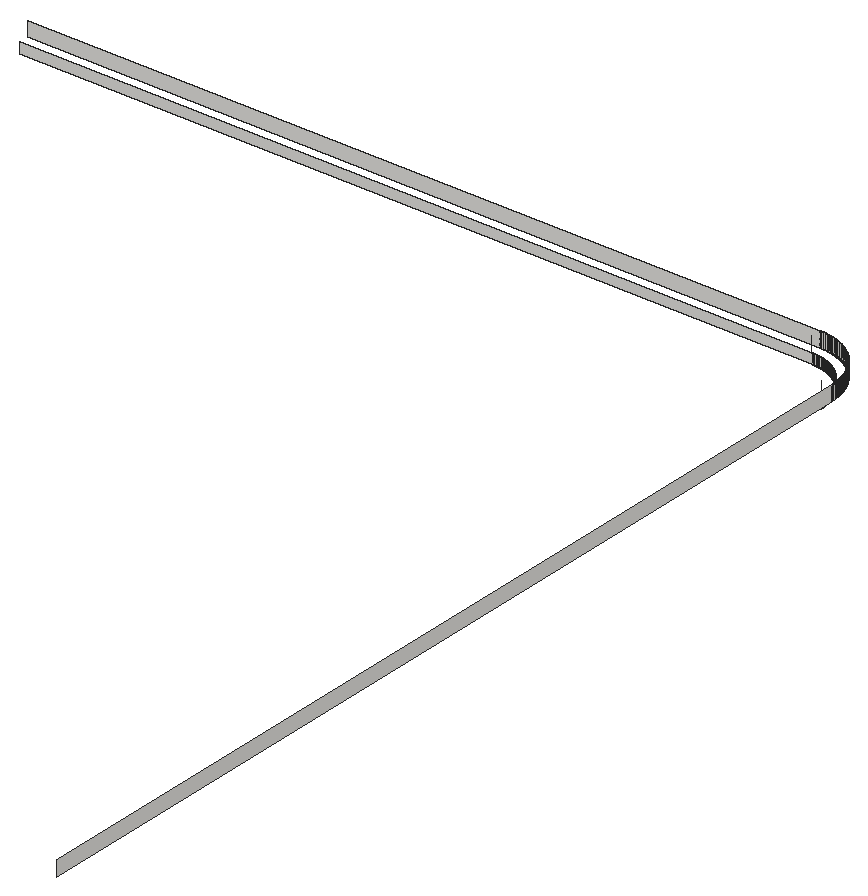
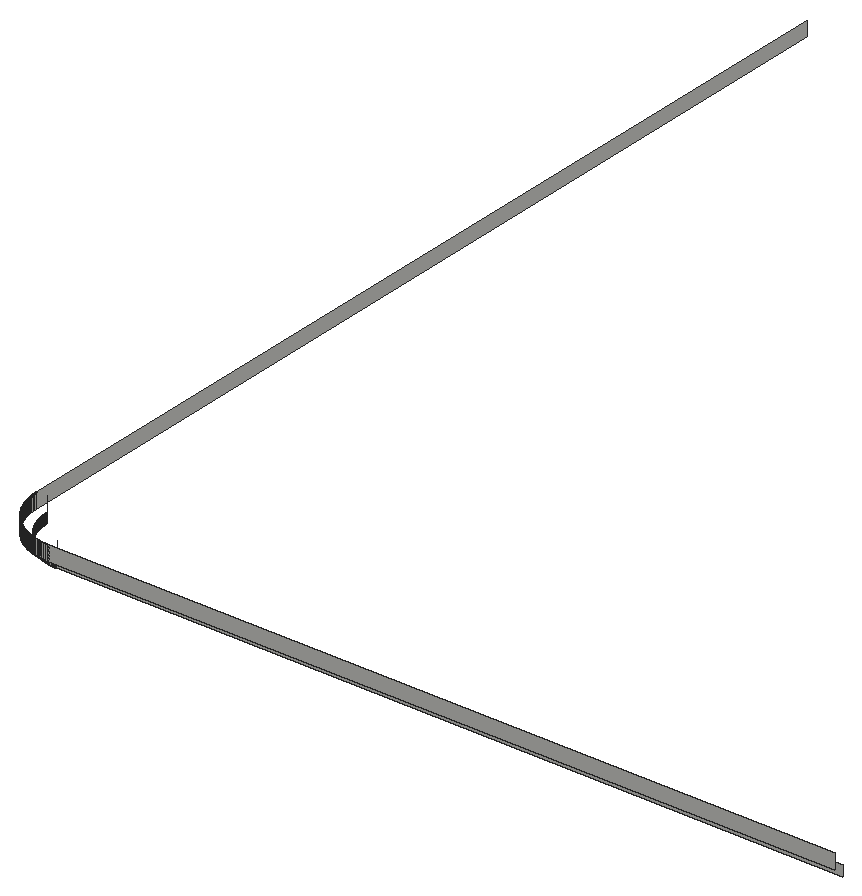
# SketchUp Ruby script. Lengths in inches.
U = 1.inch
M = Sketchup.active_model
def pt(a) = Geom::Point3d.new(a.map { |v| v * U })
def face(e, loops, mat)
  f = e.add_face(loops[0].map { |a| pt(a) })
  loops[1..].each { |l| e.add_face(l.map { |a| pt(a) }).erase! }
  f.material = f.back_material = mat if mat
  f
end
# faces: each face lists its corners as indices into pts; further lists are holes
def faces(e, pts, list, mat = nil) = list.each { |f| face(e, (f[0].is_a?(Array) ? f : [f]).map { |l| l.map { |i| pts[i] } }, mat) }
# xy, xz, yz: faces in a plane at the given z, y or x. An outline is a flat list of corners, or four numbers for a rectangle; further outlines are holes
def ring(l) = l.size == 4 ? [[l[0], l[1]], [l[2], l[1]], [l[2], l[3]], [l[0], l[3]]] : l.each_slice(2).to_a
def flat(e, list, mat, &to3) = list.each { |f| face(e, (f[0].is_a?(Array) ? f : [f]).map { |l| ring(l).map { |u, v| to3.(u, v) } }, mat) }
def xy(e, z, list, mat = nil) = flat(e, list, mat) { |x, y| [x, y, z] }
def xz(e, y, list, mat = nil) = flat(e, list, mat) { |x, z| [x, y, z] }
def yz(e, x, list, mat = nil) = flat(e, list, mat) { |y, z| [x, y, z] }
def lines(e, pts, list) = list.each { |a, b| e.add_line(pt(pts[a]), pt(pts[b])) }
# prism: a flat outline (further loops are holes) pulled along v
def prism(e, loops, v, mat = nil)
  f = face(e, loops, mat); d = Geom::Vector3d.new(v.map { |x| x * U })
  f.pushpull(f.normal.samedirection?(d) ? d.length : -d.length)
end
def box(e, o, s, mat = nil) = prism(e, [[o, [o[0] + s[0], o[1], o[2]], [o[0] + s[0], o[1] + s[1], o[2]], [o[0], o[1] + s[1], o[2]]]], [0, 0, s[2]], mat)
def at(x, y, z, deg = 0) = Geom::Transformation.translation(pt([x, y, z])) * Geom::Transformation.rotation(ORIGIN, Z_AXIS, deg.degrees)
def axes(o, x, y, z) = Geom::Transformation.new([*x, 0, *y, 0, *z, 0, *pt(o).to_a, 1])
def part(name) = M.definitions.add(name)
# library, detail: a bought-in or finely detailed component or shape, given as its bounding box
def library(name, o, s) = part(name).tap { |d| box(d.entities, o, s) }
def detail(e, o, s) = box(e.add_group.entities, o, s)
def put(e, d, t, mat = nil) = e.add_instance(d, t).tap { |i| i.material = mat if mat }
def group(e, t, mat = nil) = e.add_group.tap { |g| g.transformation = t; g.material = mat if mat }.entities
root = M.entities
M.materials.add("[Formica Graystone]").color = [224, 223, 219]
xz(root,441.99,[[174.39,422.82,174.52,424.82]],"[Formica Graystone]")
xz(root,442,[[18,422.82,174,424.82],[174,422.82,174.13,424.82],[174.13,422.82,174.26,424.82]],"[Formica Graystone]")
xz(root,444,[[18,424.82,174,427.82],[174,424.82,174.16,427.82],[174.16,424.82,174.3125,427.82]],"[Formica Graystone]")
yz(root,183.99,[[432.39,422.82,432.52,424.82]],"[Formica Graystone]")
yz(root,184,[[432,422.82,432.13,424.82],[432.13,422.82,432.26,424.82]],"[Formica Graystone]")
yz(root,186,[[241,424.82,432,427.82],[432,424.82,432.16,427.82],[432.16,424.82,432.3125,427.82]],"[Formica Graystone]")
p = [[183.99,432.39,422.82],[183.99,432.39,424.82],[184,432.26,424.82],[184,432.26,422.82],[183.98,432.65,422.82],[183.98,432.65,424.82],
  [183.99,432.52,424.82],[183.99,432.52,422.82],[183.97,432.78,422.82],[183.97,432.78,424.82],[183.96,432.92,422.82],[183.96,432.92,424.82],
  [183.95,433.05,422.82],[183.95,433.05,424.82],[183.93,433.18,422.82],[183.93,433.18,424.82],[183.91,433.31,422.82],[183.91,433.31,424.82],
  [183.9,433.43,422.82],[183.9,433.43,424.82],[183.875,433.5625,422.82],[183.875,433.5625,424.82],[183.86,433.69,422.82],[183.86,433.69,424.82],
  [183.83,433.82,422.82],[183.83,433.82,424.82],[183.81,433.95,422.82],[183.81,433.95,424.82],[183.78,434.08,422.82],[183.78,434.08,424.82],
  [183.75,434.21,422.82],[183.75,434.21,424.82],[183.72,434.33,422.82],[183.72,434.33,424.82],[183.69,434.46,422.82],[183.69,434.46,424.82],
  [183.66,434.59,422.82],[183.66,434.59,424.82],[183.625,434.71,422.82],[183.625,434.71,424.82],[183.59,434.84,422.82],[183.59,434.84,424.82],
  [183.55,434.97,422.82],[183.55,434.97,424.82],[183.51,435.09,422.82],[183.51,435.09,424.82],[183.47,435.21,422.82],[183.47,435.21,424.82],
  [183.43,435.34,422.82],[183.43,435.34,424.82],[183.38,435.46,422.82],[183.38,435.46,424.82],[183.34,435.58,422.82],[183.34,435.58,424.82],
  [183.29,435.71,422.82],[183.29,435.71,424.82],[183.24,435.83,422.82],[183.24,435.83,424.82],[183.1875,435.95,422.82],[183.1875,435.95,424.82],
  [183.14,436.07,422.82],[183.14,436.07,424.82],[183.08,436.1875,422.82],[183.08,436.1875,424.82],[183.03,436.31,422.82],[183.03,436.31,424.82],
  [182.97,436.42,422.82],[182.97,436.42,424.82],[182.91,436.54,422.82],[182.91,436.54,424.82],[182.85,436.66,422.82],[182.85,436.66,424.82],
  [182.79,436.77,422.82],[182.79,436.77,424.82],[182.72,436.89,422.82],[182.72,436.89,424.82],[182.66,437,422.82],[182.66,437,424.82],
  [182.59,437.11,422.82],[182.59,437.11,424.82],[182.53,437.22,422.82],[182.53,437.22,424.82],[182.46,437.34,422.82],[182.46,437.34,424.82],
  [182.39,437.45,422.82],[182.39,437.45,424.82],[182.31,437.56,422.82],[182.31,437.56,424.82],[182.24,437.66,422.82],[182.24,437.66,424.82],
  [182.17,437.77,422.82],[182.17,437.77,424.82],[182.09,437.88,422.82],[182.09,437.88,424.82],[182.01,437.98,422.82],[182.01,437.98,424.82],
  [181.93,438.09,422.82],[181.93,438.09,424.82],[181.85,438.19,422.82],[181.85,438.19,424.82],[181.77,438.29,422.82],[181.77,438.29,424.82],
  [181.6875,438.39,422.82],[181.6875,438.39,424.82],[181.6,438.49,422.82],[181.6,438.49,424.82],[181.52,438.59,422.82],[181.52,438.59,424.82],
  [181.43,438.69,422.82],[181.43,438.69,424.82],[181.34,438.79,422.82],[181.34,438.79,424.82],[181.25,438.88,422.82],[181.25,438.88,424.82],
  [181.16,438.98,422.82],[181.16,438.98,424.82],[181.07,439.07,422.82],[181.07,439.07,424.82],[180.98,439.16,422.82],[180.98,439.16,424.82],
  [180.88,439.25,422.82],[180.88,439.25,424.82],[180.69,439.43,422.82],[180.69,439.43,424.82],[180.79,439.34,424.82],[180.79,439.34,422.82],
  [180.59,439.52,422.82],[180.59,439.52,424.82],[180.49,439.6,422.82],[180.49,439.6,424.82],[180.39,439.6875,422.82],[180.39,439.6875,424.82],
  [180.29,439.77,422.82],[180.29,439.77,424.82],[180.19,439.85,422.82],[180.19,439.85,424.82],[179.98,440.01,422.82],[179.98,440.01,424.82],
  [180.09,439.93,424.82],[180.09,439.93,422.82],[179.88,440.09,422.82],[179.88,440.09,424.82],[179.77,440.17,422.82],[179.77,440.17,424.82],
  [179.56,440.31,422.82],[179.56,440.31,424.82],[179.66,440.24,424.82],[179.66,440.24,422.82],[179.45,440.39,422.82],[179.45,440.39,424.82],
  [179.34,440.46,422.82],[179.34,440.46,424.82],[179.11,440.59,422.82],[179.11,440.59,424.82],[179.22,440.53,424.82],[179.22,440.53,422.82],
  [179,440.66,422.82],[179,440.66,424.82],[178.77,440.79,422.82],[178.77,440.79,424.82],[178.89,440.72,424.82],[178.89,440.72,422.82],
  [178.54,440.91,422.82],[178.54,440.91,424.82],[178.66,440.85,424.82],[178.66,440.85,422.82],[178.42,440.97,422.82],[178.42,440.97,424.82],
  [178.1875,441.08,422.82],[178.1875,441.08,424.82],[178.31,441.03,424.82],[178.31,441.03,422.82],[177.95,441.1875,422.82],[177.95,441.1875,424.82],
  [178.07,441.14,424.82],[178.07,441.14,422.82],[177.71,441.29,422.82],[177.71,441.29,424.82],[177.83,441.24,424.82],[177.83,441.24,422.82],
  [177.46,441.38,422.82],[177.46,441.38,424.82],[177.58,441.34,424.82],[177.58,441.34,422.82],[177.21,441.47,422.82],[177.21,441.47,424.82],
  [177.34,441.43,424.82],[177.34,441.43,422.82],[176.97,441.55,422.82],[176.97,441.55,424.82],[177.09,441.51,424.82],[177.09,441.51,422.82],
  [176.59,441.66,422.82],[176.59,441.66,424.82],[176.71,441.625,424.82],[176.71,441.625,422.82],[176.84,441.59,424.82],[176.84,441.59,422.82],
  [176.21,441.75,422.82],[176.21,441.75,424.82],[176.33,441.72,424.82],[176.33,441.72,422.82],[176.46,441.69,424.82],[176.46,441.69,422.82],
  [175.69,441.86,422.82],[175.69,441.86,424.82],[175.82,441.83,424.82],[175.82,441.83,422.82],[175.95,441.81,424.82],[175.95,441.81,422.82],
  [176.08,441.78,424.82],[176.08,441.78,422.82],[174.92,441.96,422.82],[174.92,441.96,424.82],[175.05,441.95,424.82],[175.05,441.95,422.82],
  [175.18,441.93,424.82],[175.18,441.93,422.82],[175.31,441.91,424.82],[175.31,441.91,422.82],[175.43,441.9,424.82],[175.43,441.9,422.82],
  [175.5625,441.875,424.82],[175.5625,441.875,422.82],[174.26,442,422.82],[174.26,442,424.82],[174.39,441.99,424.82],[174.39,441.99,422.82],
  [174.52,441.99,422.82],[174.52,441.99,424.82],[174.65,441.98,424.82],[174.65,441.98,422.82],[174.78,441.97,424.82],[174.78,441.97,422.82],
  [186,432.3125,424.82],[185.99,432.47,424.82],[185.99,432.47,427.82],[186,432.3125,427.82],[185.98,432.63,424.82],[185.98,432.63,427.82],
  [185.97,432.78,424.82],[185.97,432.78,427.82],[185.96,432.94,424.82],[185.96,432.94,427.82],[185.95,433.1,424.82],[185.95,433.1,427.82],
  [185.93,433.25,424.82],[185.93,433.25,427.82],[185.92,433.41,424.82],[185.92,433.41,427.82],[185.9,433.57,424.82],[185.9,433.57,427.82],
  [185.875,433.72,424.82],[185.875,433.72,427.82],[185.85,433.88,424.82],[185.85,433.88,427.82],[185.83,434.03,424.82],[185.83,434.03,427.82],
  [185.8,434.1875,424.82],[185.8,434.1875,427.82],[185.77,434.34,424.82],[185.77,434.34,427.82],[185.74,434.49,424.82],[185.74,434.49,427.82],
  [185.7,434.65,424.82],[185.7,434.65,427.82],[185.67,434.8,424.82],[185.67,434.8,427.82],[185.63,434.95,424.82],[185.63,434.95,427.82],
  [185.59,435.11,424.82],[185.59,435.11,427.82],[185.55,435.26,424.82],[185.55,435.26,427.82],[185.51,435.41,424.82],[185.51,435.41,427.82],
  [185.46,435.56,424.82],[185.46,435.56,427.82],[185.41,435.71,424.82],[185.41,435.71,427.82],[185.36,435.86,424.82],[185.36,435.86,427.82],
  [185.3125,436.01,424.82],[185.3125,436.01,427.82],[185.26,436.15,424.82],[185.26,436.15,427.82],[185.2,436.3,424.82],[185.2,436.3,427.82],
  [185.15,436.45,424.82],[185.15,436.45,427.82],[185.09,436.59,424.82],[185.09,436.59,427.82],[185.03,436.74,424.82],[185.03,436.74,427.82],
  [184.96,436.88,424.82],[184.96,436.88,427.82],[184.9,437.02,424.82],[184.9,437.02,427.82],[184.83,437.17,424.82],[184.83,437.17,427.82],
  [184.76,437.31,424.82],[184.76,437.31,427.82],[184.69,437.45,424.82],[184.69,437.45,427.82],[184.62,437.59,424.82],[184.62,437.59,427.82],
  [184.55,437.73,424.82],[184.55,437.73,427.82],[184.47,437.86,424.82],[184.47,437.86,427.82],[184.39,438,424.82],[184.39,438,427.82],
  [184.3125,438.14,424.82],[184.3125,438.14,427.82],[184.23,438.27,424.82],[184.23,438.27,427.82],[184.15,438.4,424.82],[184.15,438.4,427.82],
  [184.0625,438.54,424.82],[184.0625,438.54,427.82],[183.98,438.67,424.82],[183.98,438.67,427.82],[183.89,438.8,424.82],[183.89,438.8,427.82],
  [183.8,438.93,424.82],[183.8,438.93,427.82],[183.71,439.05,424.82],[183.71,439.05,427.82],[183.62,439.18,424.82],[183.62,439.18,427.82],
  [183.52,439.31,424.82],[183.52,439.31,427.82],[183.42,439.43,424.82],[183.42,439.43,427.82],[183.33,439.55,424.82],[183.33,439.55,427.82],
  [183.23,439.67,424.82],[183.23,439.67,427.82],[183.125,439.79,424.82],[183.125,439.79,427.82],[183.02,439.91,424.82],[183.02,439.91,427.82],
  [182.92,440.03,424.82],[182.92,440.03,427.82],[182.8125,440.15,424.82],[182.8125,440.15,427.82],[182.7,440.26,424.82],[182.7,440.26,427.82],
  [182.6,440.375,424.82],[182.6,440.375,427.82],[182.49,440.49,424.82],[182.49,440.49,427.82],[182.375,440.6,424.82],[182.375,440.6,427.82],
  [182.26,440.7,424.82],[182.26,440.7,427.82],[182.15,440.8125,424.82],[182.15,440.8125,427.82],[182.03,440.92,424.82],[182.03,440.92,427.82],
  [181.91,441.02,424.82],[181.91,441.02,427.82],[181.79,441.125,424.82],[181.79,441.125,427.82],[181.67,441.23,424.82],[181.67,441.23,427.82],
  [181.55,441.33,424.82],[181.55,441.33,427.82],[181.43,441.42,424.82],[181.43,441.42,427.82],[181.31,441.52,424.82],[181.31,441.52,427.82],
  [181.18,441.62,424.82],[181.18,441.62,427.82],[181.05,441.71,424.82],[181.05,441.71,427.82],[180.93,441.8,424.82],[180.93,441.8,427.82],
  [180.8,441.89,424.82],[180.8,441.89,427.82],[180.67,441.98,424.82],[180.67,441.98,427.82],[180.54,442.0625,424.82],[180.54,442.0625,427.82],
  [180.4,442.15,424.82],[180.27,442.23,424.82],[180.27,442.23,427.82],[180.4,442.15,427.82],[180.14,442.3125,424.82],[180.14,442.3125,427.82],
  [180,442.39,424.82],[180,442.39,427.82],[179.86,442.47,424.82],[179.86,442.47,427.82],[179.73,442.55,424.82],[179.59,442.62,424.82],
  [179.59,442.62,427.82],[179.73,442.55,427.82],[179.45,442.69,424.82],[179.45,442.69,427.82],[179.31,442.76,424.82],[179.31,442.76,427.82],
  [179.17,442.83,424.82],[179.02,442.9,424.82],[179.02,442.9,427.82],[179.17,442.83,427.82],[178.88,442.96,424.82],[178.88,442.96,427.82],
  [178.74,443.03,424.82],[178.59,443.09,424.82],[178.59,443.09,427.82],[178.74,443.03,427.82],[178.45,443.15,424.82],[178.3,443.2,424.82],
  [178.3,443.2,427.82],[178.45,443.15,427.82],[178.15,443.26,424.82],[178.15,443.26,427.82],[178.01,443.3125,424.82],[177.86,443.36,424.82],
  [177.86,443.36,427.82],[178.01,443.3125,427.82],[177.71,443.41,424.82],[177.56,443.46,424.82],[177.56,443.46,427.82],[177.71,443.41,427.82],
  [177.26,443.55,424.82],[177.11,443.59,424.82],[177.11,443.59,427.82],[177.26,443.55,427.82],[177.41,443.51,424.82],[177.41,443.51,427.82],
  [176.95,443.63,424.82],[176.8,443.67,424.82],[176.8,443.67,427.82],[176.95,443.63,427.82],[176.49,443.74,424.82],[176.34,443.77,424.82],
  [176.34,443.77,427.82],[176.49,443.74,427.82],[176.65,443.7,424.82],[176.65,443.7,427.82],[176.03,443.83,424.82],[175.88,443.85,424.82],
  [175.88,443.85,427.82],[176.03,443.83,427.82],[176.1875,443.8,424.82],[176.1875,443.8,427.82],[175.1,443.95,424.82],[174.94,443.96,424.82],
  [174.94,443.96,427.82],[175.1,443.95,427.82],[175.25,443.93,424.82],[175.25,443.93,427.82],[175.41,443.92,424.82],[175.41,443.92,427.82],
  [175.57,443.9,424.82],[175.57,443.9,427.82],[175.72,443.875,424.82],[175.72,443.875,427.82],[174.47,443.99,424.82],[174.3125,444,424.82],
  [174.3125,444,427.82],[174.47,443.99,427.82],[174.63,443.98,424.82],[174.63,443.98,427.82],[174.78,443.97,424.82],[174.78,443.97,427.82],
  [184,432,424.82],[184,432,427.82],[174,442,424.82],[174,442,427.82]]
faces(root,p,[[0,1,2,3],[4,5,6,7],[8,9,5,4],[10,11,9,8],[12,13,11,10],[14,15,13,12],[16,17,15,14],[18,19,17,16],
  [20,21,19,18],[22,23,21,20],[24,25,23,22],[26,27,25,24],[28,29,27,26],[30,31,29,28],[32,33,31,30],[34,35,33,32],
  [36,37,35,34],[38,39,37,36],[40,41,39,38],[42,43,41,40],[44,45,43,42],[46,47,45,44],[48,49,47,46],[50,51,49,48],
  [52,53,51,50],[54,55,53,52],[56,57,55,54],[58,59,57,56],[60,61,59,58],[62,63,61,60],[64,65,63,62],[66,67,65,64],
  [68,69,67,66],[70,71,69,68],[72,73,71,70],[74,75,73,72],[76,77,75,74],[78,79,77,76],[80,81,79,78],[82,83,81,80],
  [84,85,83,82],[86,87,85,84],[88,89,87,86],[90,91,89,88],[92,93,91,90],[94,95,93,92],[96,97,95,94],[98,99,97,96],
  [100,101,99,98],[102,103,101,100],[104,105,103,102],[106,107,105,104],[108,109,107,106],[110,111,109,108],[112,113,111,110],[114,115,113,112],
  [116,117,115,114],[118,119,117,116],[120,121,119,118],[122,123,124,125],[125,124,121,120],[126,127,123,122],[128,129,127,126],[130,131,129,128],
  [132,133,131,130],[134,135,133,132],[136,137,138,139],[139,138,135,134],[140,141,137,136],[142,143,141,140],[144,145,146,147],[147,146,143,142],
  [148,149,145,144],[150,151,149,148],[152,153,154,155],[155,154,151,150],[156,157,153,152],[158,159,160,161],[161,160,157,156],[162,163,164,165],
  [165,164,159,158],[166,167,163,162],[168,169,170,171],[171,170,167,166],[172,173,174,175],[175,174,169,168],[176,177,178,179],[179,178,173,172],
  [180,181,182,183],[183,182,177,176],[184,185,186,187],[187,186,181,180],[188,189,190,191],[191,190,185,184],[192,193,194,195],[195,194,196,197],
  [197,196,189,188],[198,199,200,201],[201,200,202,203],[203,202,193,192],[204,205,206,207],[207,206,208,209],[209,208,210,211],[211,210,199,198],
  [212,213,214,215],[215,214,216,217],[217,216,218,219],[219,218,220,221],[221,220,222,223],[223,222,205,204],[224,225,226,227],[228,229,230,231],
  [231,230,232,233],[233,232,213,212],[234,235,236,237],[235,238,239,236],[238,240,241,239],[240,242,243,241],[242,244,245,243],[244,246,247,245],
  [246,248,249,247],[248,250,251,249],[250,252,253,251],[252,254,255,253],[254,256,257,255],[256,258,259,257],[258,260,261,259],[260,262,263,261],
  [262,264,265,263],[264,266,267,265],[266,268,269,267],[268,270,271,269],[270,272,273,271],[272,274,275,273],[274,276,277,275],[276,278,279,277],
  [278,280,281,279],[280,282,283,281],[282,284,285,283],[284,286,287,285],[286,288,289,287],[288,290,291,289],[290,292,293,291],[292,294,295,293],
  [294,296,297,295],[296,298,299,297],[298,300,301,299],[300,302,303,301],[302,304,305,303],[304,306,307,305],[306,308,309,307],[308,310,311,309],
  [310,312,313,311],[312,314,315,313],[314,316,317,315],[316,318,319,317],[318,320,321,319],[320,322,323,321],[322,324,325,323],[324,326,327,325],
  [326,328,329,327],[328,330,331,329],[330,332,333,331],[332,334,335,333],[334,336,337,335],[336,338,339,337],[338,340,341,339],[340,342,343,341],
  [342,344,345,343],[344,346,347,345],[346,348,349,347],[348,350,351,349],[350,352,353,351],[352,354,355,353],[354,356,357,355],[356,358,359,357],
  [358,360,361,359],[360,362,363,361],[362,364,365,363],[364,366,367,365],[366,368,369,367],[368,370,371,369],[370,372,373,371],[372,374,375,373],
  [374,376,377,375],[376,378,379,377],[378,380,381,379],[380,382,383,381],[384,385,386,387],[382,384,387,383],[385,388,389,386],[388,390,391,389],
  [390,392,393,391],[394,395,396,397],[392,394,397,393],[395,398,399,396],[398,400,401,399],[402,403,404,405],[400,402,405,401],[403,406,407,404],
  [408,409,410,411],[406,408,411,407],[412,413,414,415],[409,412,415,410],[413,416,417,414],[418,419,420,421],[416,418,421,417],[422,423,424,425],
  [419,422,425,420],[426,427,428,429],[430,426,429,431],[423,430,431,424],[432,433,434,435],[427,432,435,428],[436,437,438,439],[440,436,439,441],
  [433,440,441,434],[442,443,444,445],[446,442,445,447],[437,446,447,438],[448,449,450,451],[452,448,451,453],[454,452,453,455],[456,454,455,457],
  [458,456,457,459],[443,458,459,444],[460,461,462,463],[464,460,463,465],[466,464,465,467],[449,466,467,450]],"[Formica Graystone]")
lines(root,p,[[468,469],[470,471]])
